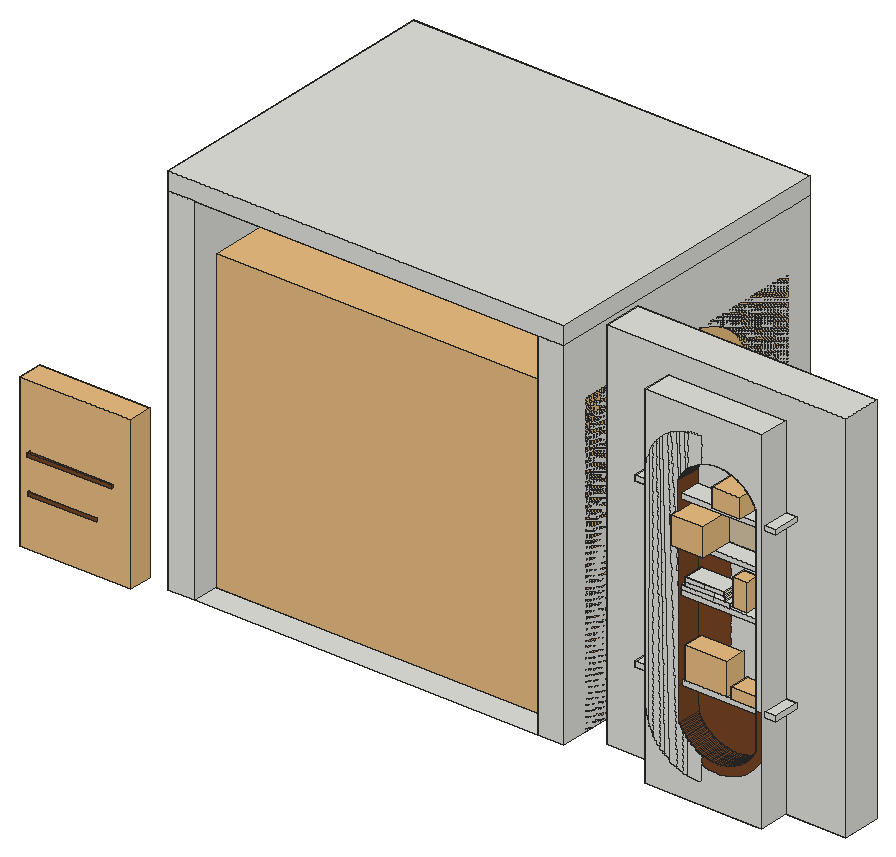
# SketchUp Ruby script. Lengths in inches.
U = 1.inch
M = Sketchup.active_model
def pt(a) = Geom::Point3d.new(a.map { |v| v * U })
def face(e, loops, mat)
  f = e.add_face(loops[0].map { |a| pt(a) })
  loops[1..].each { |l| e.add_face(l.map { |a| pt(a) }).erase! }
  f.material = f.back_material = mat if mat
  f
end
# faces: each face lists its corners as indices into pts; further lists are holes
def faces(e, pts, list, mat = nil) = list.each { |f| face(e, (f[0].is_a?(Array) ? f : [f]).map { |l| l.map { |i| pts[i] } }, mat) }
# xy, xz, yz: faces in a plane at the given z, y or x. An outline is a flat list of corners, or four numbers for a rectangle; further outlines are holes
def ring(l) = l.size == 4 ? [[l[0], l[1]], [l[2], l[1]], [l[2], l[3]], [l[0], l[3]]] : l.each_slice(2).to_a
def flat(e, list, mat, &to3) = list.each { |f| face(e, (f[0].is_a?(Array) ? f : [f]).map { |l| ring(l).map { |u, v| to3.(u, v) } }, mat) }
def xy(e, z, list, mat = nil) = flat(e, list, mat) { |x, y| [x, y, z] }
def xz(e, y, list, mat = nil) = flat(e, list, mat) { |x, z| [x, y, z] }
def yz(e, x, list, mat = nil) = flat(e, list, mat) { |y, z| [x, y, z] }
def lines(e, pts, list) = list.each { |a, b| e.add_line(pt(pts[a]), pt(pts[b])) }
# prism: a flat outline (further loops are holes) pulled along v
def prism(e, loops, v, mat = nil)
  f = face(e, loops, mat); d = Geom::Vector3d.new(v.map { |x| x * U })
  f.pushpull(f.normal.samedirection?(d) ? d.length : -d.length)
end
def box(e, o, s, mat = nil) = prism(e, [[o, [o[0] + s[0], o[1], o[2]], [o[0] + s[0], o[1] + s[1], o[2]], [o[0], o[1] + s[1], o[2]]]], [0, 0, s[2]], mat)
def at(x, y, z, deg = 0) = Geom::Transformation.translation(pt([x, y, z])) * Geom::Transformation.rotation(ORIGIN, Z_AXIS, deg.degrees)
def axes(o, x, y, z) = Geom::Transformation.new([*x, 0, *y, 0, *z, 0, *pt(o).to_a, 1])
def part(name) = M.definitions.add(name)
# library, detail: a bought-in or finely detailed component or shape, given as its bounding box
def library(name, o, s) = part(name).tap { |d| box(d.entities, o, s) }
def detail(e, o, s) = box(e.add_group.entities, o, s)
def put(e, d, t, mat = nil) = e.add_instance(d, t).tap { |i| i.material = mat if mat }
def group(e, t, mat = nil) = e.add_group.tap { |g| g.transformation = t; g.material = mat if mat }.entities
root = M.entities
M.materials.add("Douglas Fir, Staggered with Shadowgap (CXYQC8)").color = [216, 197, 167]
M.materials.add("[Color_000]").color = [255, 255, 255]
M.materials.add("[Color_D05]").color = [255, 242, 204]
M.materials.add("[Wood Veneer 01]").color = [120, 70, 37]
c1 = library("Sony_TV_KDL42W705B.skp\#1",[-24.34,-0.25,1.74],[48.68,2.34,28.26])
c2 = library("Component",[-53.76,-1.97,-0.51],[47.25,4.73,6.22])
c3 = library("Ring pendant light",[-446.05,-425.1,-51.8],[906.89,953.39,1136.48])
c4 = part("e7b7-889f-4641-7af6")
g1 = group(c4.entities,at(0,0,0))
g2 = group(g1,at(0,0,0))
put(g2,c3,axes([0,0,0],[39.37008,0,0],[0,39.37008,0],[0,0,39.37008]))
c5 = library("Plant_pot\#1",[-1.14,-1.38,0],[9.4,9.4,6.47])
c6 = library("Books+01+VRAY+ready",[65.64,68.87,0],[14.63,11.84,5.35])
c7 = part("Hardcover book")
xy(c7.entities,0,[[0.12,0.12,1.11,7.49]])
xy(c7.entities,0,[[0,0,0,7.57,0.12,7.57,0.12,0.12,1.11,0.12,1.11,7.57,1.22,7.57,1.22,0]],"[Color_000]")
xy(c7.entities,9.7,[[0.12,0.13,1.11,7.51]],"[Color_D05]")
xy(c7.entities,9.81,[[0,0.02,1.22,0.02,1.22,7.59,1.11,7.59,1.11,0.13,0.12,0.13,0.12,7.59,0,7.59]],"[Color_000]")
xz(c7.entities,0.13,[[0.12,9.7,1.11,9.81]],"[Color_000]")
yz(c7.entities,0,[[0,0,0.01,7.28,0.02,9.81,7.59,9.81,7.57,0]],"[Color_000]")
yz(c7.entities,0.12,[[0.12,0,7.49,0,7.51,9.7,0.13,9.7]])
yz(c7.entities,0.12,[[7.49,0,7.57,0,7.59,9.81,0.13,9.81,0.13,9.7,7.51,9.7]],"[Color_000]")
yz(c7.entities,1.11,[[0.12,0,0.13,9.7,7.51,9.7,7.49,0]])
yz(c7.entities,1.11,[[7.49,0,7.51,9.7,0.13,9.7,0.13,9.81,7.59,9.81,7.57,0]],"[Color_000]")
yz(c7.entities,1.22,[[0,0,7.57,0,7.59,9.81,0.02,9.81,0.01,7.28]])
p = [[1.22,0,0],[1.22,0.01,7.28],[0,0.01,7.28],[0,0,0],[1.11,0.12,0],[0.12,0.12,0],
  [0.12,0.13,9.7],[1.11,0.13,9.7],[1.11,7.49,0],[0.12,7.49,0],[0.12,7.51,9.7],[1.11,7.51,9.7],
  [0.12,7.57,0],[0,7.57,0],[0,7.59,9.81],[0.12,7.59,9.81],[1.22,7.57,0],[1.11,7.57,0],
  [1.11,7.59,9.81],[1.22,7.59,9.81],[0,0.02,9.81],[1.22,0.02,9.81]]
faces(c7.entities,p,[[0,1,2,3],[4,5,6,7],[12,13,14,15]])
faces(c7.entities,p,[[8,9,10,11]],"[Color_D05]")
faces(c7.entities,p,[[16,17,18,19],[20,2,1,21]],"[Color_000]")
c8 = part("Hardcover book \#1")
xy(c8.entities,0,[[0.12,0.12,1.11,6.86]])
xy(c8.entities,0,[[0,0,0,6.94,0.12,6.94,0.12,0.12,1.11,0.12,1.11,6.94,1.22,6.94,1.22,0]],"[Color_000]")
xy(c8.entities,9.46,[[0.12,0.13,1.11,6.88]],"[Color_D05]")
xy(c8.entities,9.57,[[0,0.02,1.22,0.02,1.22,6.96,1.11,6.96,1.11,0.13,0.12,0.13,0.12,6.96,0,6.96]],"[Color_000]")
xz(c8.entities,0.13,[[0.12,9.46,1.11,9.57]],"[Color_000]")
yz(c8.entities,0,[[0,0,0.01,4.79,0.02,9.57,6.96,9.57,6.94,0]])
yz(c8.entities,0.12,[[0.12,0,6.86,0,6.88,9.46,0.13,9.46]])
yz(c8.entities,0.12,[[6.86,0,6.94,0,6.96,9.57,0.13,9.57,0.13,9.46,6.88,9.46]],"[Color_000]")
yz(c8.entities,1.11,[[0.12,0,0.13,9.46,6.88,9.46,6.86,0]])
yz(c8.entities,1.11,[[6.86,0,6.88,9.46,0.13,9.46,0.13,9.57,6.96,9.57,6.94,0]],"[Color_000]")
yz(c8.entities,1.22,[[0,0,6.94,0,6.96,9.57,0.02,9.57,0.01,4.79]])
p = [[1.22,0,0],[1.22,0.01,4.79],[0,0.01,4.79],[0,0,0],[1.11,0.12,0],[0.12,0.12,0],
  [0.12,0.13,9.46],[1.11,0.13,9.46],[0.12,6.94,0],[0,6.94,0],[0,6.96,9.57],[0.12,6.96,9.57],
  [1.11,6.86,0],[0.12,6.86,0],[0.12,6.88,9.46],[1.11,6.88,9.46],[1.22,6.94,0],[1.11,6.94,0],
  [1.11,6.96,9.57],[1.22,6.96,9.57],[0,0.02,9.57],[1.22,0.02,9.57]]
faces(c8.entities,p,[[0,1,2,3],[4,5,6,7],[8,9,10,11],[20,2,1,21]])
faces(c8.entities,p,[[12,13,14,15]],"[Color_D05]")
faces(c8.entities,p,[[16,17,18,19]],"[Color_000]")
c9 = part("Hardcover book \#2")
xy(c9.entities,0,[[0.12,0.12,1.11,8.02]])
xy(c9.entities,0,[[0,0,0,8.1,0.12,8.1,0.12,0.12,1.11,0.12,1.11,8.1,1.22,8.1,1.22,0]],"[Color_000]")
xy(c9.entities,11.98,[[0.12,0.12,1.11,8.02]],"[Color_D05]")
xy(c9.entities,12.09,[[0,0,1.22,0,1.22,8.1,1.11,8.1,1.11,0.12,0.12,0.12,0.12,8.1,0,8.1]],"[Color_000]")
xz(c9.entities,0,[[0,0,1.22,7.96],[0,7.96,1.22,12.09]])
xz(c9.entities,0.12,[[0.12,0,1.11,11.98]])
xz(c9.entities,0.12,[[0.12,11.98,1.11,12.09]],"[Color_000]")
xz(c9.entities,8.02,[[0.12,0,1.11,11.98]],"[Color_D05]")
xz(c9.entities,8.1,[[0,0,0.12,12.09]])
xz(c9.entities,8.1,[[1.11,0,1.22,12.09]],"[Color_000]")
yz(c9.entities,0,[[0,0,8.1,12.09]])
yz(c9.entities,0.12,[[0.12,0,8.02,11.98]])
yz(c9.entities,0.12,[[8.02,0,8.1,0,8.1,12.09,0.12,12.09,0.12,11.98,8.02,11.98]],"[Color_000]")
yz(c9.entities,1.11,[[0.12,0,8.02,11.98]])
yz(c9.entities,1.11,[[8.02,0,8.02,11.98,0.12,11.98,0.12,12.09,8.1,12.09,8.1,0]],"[Color_000]")
yz(c9.entities,1.22,[[0,0,8.1,12.09]])
c10 = part("Stacked books")
put(c10.entities,c7,axes([15.01,10.96,2.78],[0,0,-1.13702],[0,-1.3536,0],[-1.3536,0,0]))
put(c10.entities,c8,axes([15.01,10.96,4.17],[0,0,-1.13702],[0,-1.3536,0],[-1.3536,0,0]))
put(c10.entities,c9,axes([16.36,10.96,1.39],[0,0,-1.13702],[0,-1.3536,0],[-1.3536,0,0]))
c11 = library("APARADOR+DE+LIVROS+CACHORRO",[95.16,10.21,2.45],[14.14,8.65,10.65])
c12 = library("Pot plante",[0,0,0],[98.24,106.18,82.98])
c13 = library("Group\#1",[0,0,0],[37,8,51])
c14 = library("Group\#10",[0,0,0],[110.17,20.41,51.91])
c15 = part("Group\#15")
box(c15.entities,[0,0,0],[47,9,1.66])
c16 = library("Group\#37",[0,0,0],[8.83,8.83,17.16])
detail(root,[42.01,15.87,0],[133,85,100.3125])
put(root,c1,at(104.17,100.77,52.78))
put(root,c2,axes([58.04,92.16,45.17],[0,0,-1],[-1,0,0],[0,1,0]))
put(root,c2,axes([156.21,94.16,49.36],[0,0,-1],[-1,0,0],[0,1,0]))
put(root,c4,axes([107.8,50.28,93.98],[0.00058,0,0],[0,0.00058,0],[0,0,0.00058]))
put(root,c5,at(228.14,5.31,90.75))
put(root,c6,axes([189.51,-39.46,34.75],[0.65,0,0],[0,0.65,0],[0,0,0.65]))
put(root,c10,at(231.86,16.27,61.75,-180))
put(root,c11,at(121.49,-4.9,32.31))
put(root,c12,axes([215.1875,1.31,76.7],[0.11,0,0],[0,0.11,0],[0,0,0.11]))
put(root,c13,at(-2.75,1,0))
g3 = group(root,at(0.2,0,28.33),"[Wood Veneer 01]")
prism(g3,[[[27.99,5.5625,0],[28.09,0.5625,0],[0.1,0,0],[0,5,0]]],[0,0,1.23])
g4 = group(root,at(-5.01,0.4375,16.27),"[Wood Veneer 01]")
xy(g4,0,[[5.1,0.1,5.01,4.56,28.01,5.02,28.09,0.5625]])
xy(g4,1.23,[[5.1,0.1,29.42,0.59,29.33,5.05,28.01,5.02,5.01,4.56]])
p = [[5.01,4.56,1.23],[5.01,4.56,0],[5.1,0.1,0],[5.1,0.1,1.23],[28.09,0.5625,0],[29.42,0.59,0],
  [29.42,0.59,1.23],[28.01,5.02,0],[28.01,5.02,1.23],[29.33,5.05,1.23]]
faces(g4,p,[[0,1,2,3],[2,4,5,6,3],[7,8,4],[4,8,9,5],[6,5,9],[8,7,1,0]])
g5 = group(root,at(166.01,6.87,0))
xy(g5,0,[[0,0,9,29.67],[0,77.14,9,103]])
xy(g5,120,[[0,0,9,103]])
xz(g5,0,[[0,0,9,120]])
xz(g5,29.67,[[0,0,9,82.3125]])
xz(g5,77.14,[[0,0,9,82.3125]])
xz(g5,103,[[0,0,9,120]])
yz(g5,0,[[0,0,0,120,94,120,94,0,77.14,0,77.14,82.3125,76.91,83.08,76.66,83.84,76.38,84.59,76.08,85.33,75.76,86.06,75.41,86.78,75.04,87.49,74.64,88.18,74.22,88.86,73.78,89.53,73.32,90.1875,72.84,90.82,72.34,91.45,71.82,92.05,71.28,92.64,70.72,93.21,70.14,93.76,69.54,94.3,68.93,94.8125,68.3,95.3,67.66,95.78,67,96.23,66.32,96.66,65.63,97.07,64.93,97.45,64.22,97.8125,63.5,98.15,62.76,98.47,62.02,98.76,61.26,99.03,60.5,99.27,59.73,99.49,58.95,99.68,58.17,99.85,57.39,99.99,56.59,100.11,55.8,100.2,55,100.26,54.2,100.3,53.4,100.3125,52.61,100.3,51.81,100.26,51.01,100.2,50.22,100.11,49.42,99.99,48.64,99.85,47.86,99.68,47.08,99.49,46.31,99.27,45.55,99.03,44.79,98.76,44.05,98.47,43.3125,98.15,42.59,97.8125,41.88,97.45,41.18,97.07,40.49,96.66,39.81,96.23,39.15,95.78,38.51,95.3,37.88,94.8125,37.27,94.3,36.67,93.76,36.09,93.21,35.53,92.64,34.99,92.05,34.47,91.45,33.97,90.82,33.49,90.1875,33.03,89.53,32.59,88.86,32.17,88.18,31.77,87.49,31.4,86.78,31.05,86.06,30.73,85.33,30.43,84.59,30.15,83.84,29.9,83.08,29.67,82.3125,29.67,0],[94,0,103,120]])
yz(g5,9,[[0,0,29.67,0,29.67,82.3125,29.9,83.08,30.15,83.84,30.43,84.59,30.73,85.33,31.05,86.06,31.4,86.78,31.77,87.49,32.17,88.18,32.59,88.86,33.03,89.53,33.49,90.1875,33.97,90.82,34.47,91.45,34.99,92.05,35.53,92.64,36.09,93.21,36.67,93.76,37.27,94.3,37.88,94.8125,38.51,95.3,39.15,95.78,39.81,96.23,40.49,96.66,41.18,97.07,41.88,97.45,42.59,97.8125,43.3125,98.15,44.05,98.47,44.79,98.76,45.55,99.03,46.31,99.27,47.08,99.49,47.86,99.68,48.64,99.85,49.42,99.99,50.22,100.11,51.01,100.2,51.81,100.26,52.61,100.3,53.4,100.3125,54.2,100.3,55,100.26,55.8,100.2,56.59,100.11,57.39,99.99,58.17,99.85,58.95,99.68,59.73,99.49,60.5,99.27,61.26,99.03,62.02,98.76,62.76,98.47,63.5,98.15,64.22,97.8125,64.93,97.45,65.63,97.07,66.32,96.66,67,96.23,67.66,95.78,68.3,95.3,68.93,94.8125,69.54,94.3,70.14,93.76,70.72,93.21,71.28,92.64,71.82,92.05,72.34,91.45,72.84,90.82,73.32,90.1875,73.78,89.53,74.22,88.86,74.64,88.18,75.04,87.49,75.41,86.78,75.76,86.06,76.08,85.33,76.38,84.59,76.66,83.84,76.91,83.08,77.14,82.3125,77.14,0,103,0,103,120,0,120]])
p = [[0,29.67,82.3125],[0,29.9,83.08],[9,29.9,83.08],[9,29.67,82.3125],[0,76.91,83.08],[0,77.14,82.3125],
  [9,77.14,82.3125],[9,76.91,83.08],[0,30.15,83.84],[9,30.15,83.84],[0,76.66,83.84],[9,76.66,83.84],
  [0,30.43,84.59],[9,30.43,84.59],[0,76.38,84.59],[9,76.38,84.59],[0,30.73,85.33],[9,30.73,85.33],
  [0,76.08,85.33],[9,76.08,85.33],[0,31.05,86.06],[9,31.05,86.06],[0,75.76,86.06],[9,75.76,86.06],
  [0,31.4,86.78],[9,31.4,86.78],[0,75.41,86.78],[9,75.41,86.78],[0,31.77,87.49],[9,31.77,87.49],
  [0,75.04,87.49],[9,75.04,87.49],[0,32.17,88.18],[9,32.17,88.18],[0,74.64,88.18],[9,74.64,88.18],
  [0,32.59,88.86],[9,32.59,88.86],[0,74.22,88.86],[9,74.22,88.86],[0,33.03,89.53],[9,33.03,89.53],
  [0,73.78,89.53],[9,73.78,89.53],[0,33.49,90.1875],[9,33.49,90.1875],[0,73.32,90.1875],[9,73.32,90.1875],
  [0,33.97,90.82],[9,33.97,90.82],[0,72.84,90.82],[9,72.84,90.82],[0,34.47,91.45],[9,34.47,91.45],
  [0,72.34,91.45],[9,72.34,91.45],[0,34.99,92.05],[9,34.99,92.05],[0,71.82,92.05],[9,71.82,92.05],
  [0,35.53,92.64],[9,35.53,92.64],[0,71.28,92.64],[9,71.28,92.64],[0,36.09,93.21],[9,36.09,93.21],
  [0,70.72,93.21],[9,70.72,93.21],[0,36.67,93.76],[9,36.67,93.76],[0,70.14,93.76],[9,70.14,93.76],
  [0,37.27,94.3],[9,37.27,94.3],[0,69.54,94.3],[9,69.54,94.3],[0,37.88,94.8125],[9,37.88,94.8125],
  [0,68.93,94.8125],[9,68.93,94.8125],[0,38.51,95.3],[9,38.51,95.3],[0,68.3,95.3],[9,68.3,95.3],
  [0,39.15,95.78],[9,39.15,95.78],[0,67.66,95.78],[9,67.66,95.78],[0,39.81,96.23],[9,39.81,96.23],
  [0,67,96.23],[9,67,96.23],[0,40.49,96.66],[9,40.49,96.66],[0,66.32,96.66],[9,66.32,96.66],
  [0,41.18,97.07],[9,41.18,97.07],[0,65.63,97.07],[9,65.63,97.07],[0,41.88,97.45],[9,41.88,97.45],
  [0,64.93,97.45],[9,64.93,97.45],[0,42.59,97.8125],[9,42.59,97.8125],[0,64.22,97.8125],[9,64.22,97.8125],
  [0,43.3125,98.15],[9,43.3125,98.15],[0,63.5,98.15],[9,63.5,98.15],[0,44.05,98.47],[9,44.05,98.47],
  [0,62.76,98.47],[9,62.76,98.47],[0,44.79,98.76],[9,44.79,98.76],[0,62.02,98.76],[9,62.02,98.76],
  [0,45.55,99.03],[9,45.55,99.03],[0,61.26,99.03],[9,61.26,99.03],[0,46.31,99.27],[9,46.31,99.27],
  [0,60.5,99.27],[9,60.5,99.27],[0,47.08,99.49],[9,47.08,99.49],[0,59.73,99.49],[9,59.73,99.49],
  [0,47.86,99.68],[9,47.86,99.68],[0,58.95,99.68],[9,58.95,99.68],[0,48.64,99.85],[9,48.64,99.85],
  [0,58.17,99.85],[9,58.17,99.85],[0,49.42,99.99],[9,49.42,99.99],[0,57.39,99.99],[9,57.39,99.99],
  [0,50.22,100.11],[9,50.22,100.11],[0,56.59,100.11],[9,56.59,100.11],[0,51.01,100.2],[9,51.01,100.2],
  [0,55.8,100.2],[9,55.8,100.2],[0,51.81,100.26],[9,51.81,100.26],[0,55,100.26],[9,55,100.26],
  [0,52.61,100.3],[9,52.61,100.3],[0,53.4,100.3125],[9,53.4,100.3125],[0,54.2,100.3],[9,54.2,100.3]]
faces(g5,p,[[0,1,2,3],[4,5,6,7],[1,8,9,2],[10,4,7,11],[8,12,13,9],[14,10,11,15],[12,16,17,13],[18,14,15,19],
  [16,20,21,17],[22,18,19,23],[20,24,25,21],[26,22,23,27],[24,28,29,25],[30,26,27,31],[28,32,33,29],[34,30,31,35],
  [32,36,37,33],[38,34,35,39],[36,40,41,37],[42,38,39,43],[40,44,45,41],[46,42,43,47],[44,48,49,45],[50,46,47,51],
  [48,52,53,49],[54,50,51,55],[52,56,57,53],[58,54,55,59],[56,60,61,57],[62,58,59,63],[60,64,65,61],[66,62,63,67],
  [64,68,69,65],[70,66,67,71],[68,72,73,69],[74,70,71,75],[72,76,77,73],[78,74,75,79],[76,80,81,77],[82,78,79,83],
  [80,84,85,81],[86,82,83,87],[84,88,89,85],[90,86,87,91],[88,92,93,89],[94,90,91,95],[92,96,97,93],[98,94,95,99],
  [96,100,101,97],[102,98,99,103],[100,104,105,101],[106,102,103,107],[104,108,109,105],[110,106,107,111],[108,112,113,109],[114,110,111,115],
  [112,116,117,113],[118,114,115,119],[116,120,121,117],[122,118,119,123],[120,124,125,121],[126,122,123,127],[124,128,129,125],[130,126,127,131],
  [128,132,133,129],[134,130,131,135],[132,136,137,133],[138,134,135,139],[136,140,141,137],[142,138,139,143],[140,144,145,141],[146,142,143,147],
  [144,148,149,145],[150,146,147,151],[148,152,153,149],[154,150,151,155],[152,156,157,153],[156,158,159,157],[158,160,161,159],[160,154,155,161]])
g6 = group(root,at(51.01,6.87,0))
xy(g6,0,[[0,0,115,9]])
g7 = group(root,at(42.01,6.87,0))
prism(g7,[[[9,25.2,0],[9,25.2,82.3125],[9,25.43,83.08],[9,25.68,83.84],[9,25.96,84.59],[9,26.26,85.33],[9,26.58,86.06],[9,26.93,86.78],[9,27.3,87.49],[9,27.7,88.18],[9,28.12,88.86],[9,28.56,89.53],[9,29.02,90.1875],[9,29.5,90.82],[9,30,91.45],[9,30.52,92.05],[9,31.0625,92.64],[9,31.625,93.21],[9,32.2,93.76],[9,32.8,94.3],[9,33.41,94.8125],[9,34.04,95.3],[9,34.69,95.78],[9,35.35,96.23],[9,36.02,96.66],[9,36.71,97.07],[9,37.41,97.45],[9,38.12,97.8125],[9,38.84,98.15],[9,39.58,98.47],[9,40.32,98.76],[9,41.08,99.03],[9,41.84,99.27],[9,42.61,99.49],[9,43.39,99.68],[9,44.17,99.85],[9,44.95,99.99],[9,45.75,100.11],[9,46.54,100.2],[9,47.34,100.26],[9,48.14,100.3],[9,48.9375,100.3125],[9,49.74,100.3],[9,50.53,100.26],[9,51.33,100.2],[9,52.125,100.11],[9,52.92,99.99],[9,53.7,99.85],[9,54.49,99.68],[9,55.26,99.49],[9,56.03,99.27],[9,56.79,99.03],[9,57.55,98.76],[9,58.29,98.47],[9,59.03,98.15],[9,59.75,97.8125],[9,60.46,97.45],[9,61.16,97.07],[9,61.85,96.66],[9,62.53,96.23],[9,63.1875,95.78],[9,63.83,95.3],[9,64.46,94.8125],[9,65.07,94.3],[9,65.67,93.76],[9,66.25,93.21],[9,66.81,92.64],[9,67.35,92.05],[9,67.87,91.45],[9,68.37,90.82],[9,68.85,90.1875],[9,69.31,89.53],[9,69.75,88.86],[9,70.17,88.18],[9,70.57,87.49],[9,70.9375,86.78],[9,71.29,86.06],[9,71.61,85.33],[9,71.91,84.59],[9,72.19,83.84],[9,72.44,83.08],[9,72.67,82.3125],[9,72.67,0],[9,103,0],[9,103,120],[9,0,120],[9,0,0]]],[-9,0,0])
g8 = group(root,at(51.01,100.87,0))
xy(g8,0,[[0,-1,1.83,0],[3,-1,4.83,0],[6,-1,7.83,0],[9,-1,10.83,0],[12,-1,13.83,0],
  [15,-1,16.83,0],[95.17,-1,97,0],[98.17,-1,100,0],[101.17,-1,103,0],[104.17,-1,106,0],
  [107.17,-1,109,0],[110.17,-1,112,0],[113.17,-1,115,0],[0,0,0,9,115,9,115,0,95.17,0,95.17,2,16.83,2,16.83,0]])
xy(g8,120,[[0,-1,1.83,0],[3,-1,4.83,0],[6,-1,7.83,0],[9,-1,10.83,0],[12,-1,13.83,0],
  [15,-1,16.83,0],[95.17,-1,97,0],[98.17,-1,100,0],[101.17,-1,103,0],[104.17,-1,106,0],
  [107.17,-1,109,0],[110.17,-1,112,0],[113.17,-1,115,0],[0,0,16.83,0,16.83,2,95.17,2,95.17,0,115,0,115,9,0,9]])
xz(g8,-1,[[0,0,1.83,120],[3,0,4.83,120],[6,0,7.83,120],[9,0,10.83,120],[12,0,13.83,120],
  [15,0,16.83,120],[95.17,0,97,120],[98.17,0,100,120],[101.17,0,103,120],[104.17,0,106,120],
  [107.17,0,109,120],[110.17,0,112,120],[113.17,0,115,120]])
xz(g8,0,[[0,0,1.83,120],[1.83,0,3,120],[3,0,4.83,120],[4.83,0,6,120],[6,0,7.83,120],
  [7.83,0,9,120],[9,0,10.83,120],[10.83,0,12,120],[12,0,13.83,120],[13.83,0,15,120],
  [15,0,16.83,120],[95.17,0,97,120],[97,0,98.17,120],[98.17,0,100,120],[100,0,101.17,120],
  [101.17,0,103,120],[103,0,104.17,120],[104.17,0,106,120],[106,0,107.17,120],[107.17,0,109,120],
  [109,0,110.17,120],[110.17,0,112,120],[112,0,113.17,120],[113.17,0,115,120]])
xz(g8,2,[[16.83,0,95.17,0,95.17,120,81.5,120,81.5,28,80.5,28,80.5,120,70.5,120,70.5,28,69.5,28,69.5,120,40.5,120,40.5,28,39.5,28,39.5,120,29.5,120,29.5,28,28.5,28,28.5,120,16.83,120],[28.5,28,29.5,120],[39.5,28,40.5,120],[69.5,28,70.5,120],[80.5,28,81.5,120]])
xz(g8,9,[[0,0,115,120]])
yz(g8,0,[[-1,0,0,120],[0,0,9,120]])
yz(g8,1.83,[[-1,0,0,120]])
yz(g8,3,[[-1,0,0,120]])
yz(g8,4.83,[[-1,0,0,120]])
yz(g8,6,[[-1,0,0,120]])
yz(g8,7.83,[[-1,0,0,120]])
yz(g8,9,[[-1,0,0,120]])
yz(g8,10.83,[[-1,0,0,120]])
yz(g8,12,[[-1,0,0,120]])
yz(g8,13.83,[[-1,0,0,120]])
yz(g8,15,[[-1,0,0,120]])
yz(g8,16.83,[[-1,0,0,120],[0,0,2,120]])
yz(g8,95.17,[[-1,0,0,120],[0,0,2,120]])
yz(g8,97,[[-1,0,0,120]])
yz(g8,98.17,[[-1,0,0,120]])
yz(g8,100,[[-1,0,0,120]])
yz(g8,101.17,[[-1,0,0,120]])
yz(g8,103,[[-1,0,0,120]])
yz(g8,104.17,[[-1,0,0,120]])
yz(g8,106,[[-1,0,0,120]])
yz(g8,107.17,[[-1,0,0,120]])
yz(g8,109,[[-1,0,0,120]])
yz(g8,110.17,[[-1,0,0,120]])
yz(g8,112,[[-1,0,0,120]])
yz(g8,113.17,[[-1,0,0,120]])
yz(g8,115,[[-1,0,0,120],[0,0,9,120]])
put(root,c14,at(52.85,84.85,11.96))
g9 = group(root,at(42.01,6.87,120))
xy(g9,-1,[[64.28,17.43,63.34,17.53,62.38,17.73,61.38,18.06,60.33,18.52,59.23,19.15,58.09,19.9375,56.93,20.91,55.76,22.08,54.61,23.4375,53.48,24.98,52.41,26.71,51.4,28.61,50.48,30.67,49.66,32.86,48.96,35.18,48.38,37.6,47.9375,40.11,47.64,42.67,47.48,45.27,47.47,47.875,47.6,50.48,47.89,53.05,48.31,55.56,48.87,57.99,49.55,60.33,50.36,62.54,51.26,64.62,52.26,66.54,53.32,68.3,54.44,69.87,55.6,71.26,56.77,72.45,57.93,73.45,59.07,74.27,60.17,74.91,61.23,75.4,62.24,75.75,63.21,75.97,64.15,76.08,65.07,76.08,66.01,75.99,66.97,75.78,67.97,75.46,69.03,74.99,70.12,74.37,71.26,73.58,72.42,72.6,73.59,71.4375,74.75,70.08,75.87,68.54,76.95,66.81,77.95,64.91,78.87,62.85,79.6875,60.65,80.39,58.33,80.97,55.91,81.41,53.41,81.72,50.85,81.875,48.25,81.88,45.64,81.75,43.04,81.47,40.47,81.04,37.96,80.48,35.53,79.8,33.19,79,30.98,78.09,28.9,77.1,26.97,76.03,25.22,74.91,23.65,73.76,22.26,72.59,21.07,71.42,20.07,70.28,19.25,69.18,18.6,68.12,18.12,67.11,17.77,66.15,17.55,65.21,17.44]])
xy(g9,0,[[[0,0,133,103],[63.63,3.46,66.08,3.48,68.52,3.76,70.9375,4.3125,73.31,5.125,75.64,6.2,77.9,7.52,80.07,9.08,82.16,10.87,84.13,12.89,85.98,15.11,87.71,17.53,89.29,20.13,90.72,22.89,91.98,25.8,93.08,28.84,94.01,31.99,94.75,35.23,95.31,38.55,95.68,41.91,95.86,45.3,95.84,48.7,95.64,52.09,95.24,55.45,94.66,58.76,93.89,61.98,92.9375,65.12,91.8125,68.14,90.52,71.03,89.07,73.77,87.47,76.35,85.72,78.74,83.85,80.9375,81.86,82.92,79.77,84.68,77.58,86.21,75.31,87.49,72.97,88.53,70.59,89.3,68.17,89.8125,65.72,90.0625,63.27,90.04,60.83,89.76,58.42,89.2,56.04,88.39,53.71,87.32,51.45,86,49.28,84.44,47.2,82.65,45.22,80.63,43.37,78.41,41.65,75.99,40.07,73.39,38.64,70.625,37.37,67.72,36.27,64.68,35.34,61.53,34.6,58.28,34.04,54.97,33.67,51.61,33.49,48.22,33.51,44.8125,33.71,41.42,34.11,38.07,34.7,34.76,35.47,31.53,36.42,28.4,37.54,25.375,38.83,22.48,40.28,19.74,41.89,17.17,43.63,14.78,45.5,12.58,47.49,10.6,49.59,8.84,51.77,7.31,54.04,6.03,56.38,4.99,58.76,4.22,61.18,3.7]],[[63.63,3.46,61.18,3.7,58.76,4.22,56.38,4.99,54.04,6.03,51.77,7.31,49.59,8.84,47.49,10.6,45.5,12.58,43.63,14.78,41.89,17.17,40.28,19.74,38.83,22.48,37.54,25.375,36.42,28.4,35.47,31.53,34.7,34.76,34.11,38.07,33.71,41.42,33.51,44.8125,33.49,48.22,33.67,51.61,34.04,54.97,34.6,58.28,35.34,61.53,36.27,64.68,37.37,67.72,38.64,70.625,40.07,73.39,41.65,75.99,43.37,78.41,45.22,80.63,47.2,82.65,49.28,84.44,51.45,86,53.71,87.32,56.04,88.39,58.42,89.2,60.83,89.76,63.27,90.04,65.72,90.0625,68.17,89.8125,70.59,89.3,72.97,88.53,75.31,87.49,77.58,86.21,79.77,84.68,81.86,82.92,83.85,80.9375,85.72,78.74,87.47,76.35,89.07,73.77,90.52,71.03,91.8125,68.14,92.9375,65.12,93.89,61.98,94.66,58.76,95.24,55.45,95.64,52.09,95.84,48.7,95.86,45.3,95.68,41.91,95.31,38.55,94.75,35.23,94.01,31.99,93.08,28.84,91.98,25.8,90.72,22.89,89.29,20.13,87.71,17.53,85.98,15.11,84.13,12.89,82.16,10.87,80.07,9.08,77.9,7.52,75.64,6.2,73.31,5.125,70.9375,4.3125,68.52,3.76,66.08,3.48],[63.6875,4.76,66,4.78,68.3,5.05,70.58,5.57,72.83,6.34,75.04,7.35,77.1875,8.61,79.27,10.1,81.26,11.82,83.16,13.76,84.95,15.91,86.62,18.25,88.15,20.77,89.54,23.45,90.77,26.28,91.85,29.25,92.75,32.32,93.47,35.49,94.02,38.73,94.38,42.02,94.56,45.33,94.54,48.66,94.34,51.98,93.95,55.26,93.38,58.49,92.63,61.64,91.7,64.7,90.61,67.65,89.35,70.46,87.9375,73.125,86.39,75.62,84.7,77.93,82.9,80.05,80.98,81.96,78.97,83.65,76.88,85.11,74.72,86.33,72.51,87.31,70.25,88.04,67.97,88.53,65.66,88.76,63.36,88.74,61.05,88.47,58.77,87.95,56.52,87.18,54.3125,86.17,52.16,84.91,50.08,83.42,48.09,81.7,46.1875,79.76,44.4,77.61,42.73,75.27,41.2,72.75,39.8125,70.07,38.58,67.23,37.51,64.27,36.6,61.2,35.88,58.03,35.33,54.79,34.97,51.5,34.8,48.18,34.81,44.86,35.01,41.54,35.4,38.26,35.97,35.03,36.72,31.875,37.65,28.8125,38.75,25.87,40,23.06,41.41,20.39,42.97,17.9,44.65,15.58,46.46,13.47,48.37,11.56,50.38,9.87,52.47,8.41,54.63,7.19,56.84,6.21,59.1,5.48,61.39,4.99]],[[63.6875,4.76,61.39,4.99,59.1,5.48,56.84,6.21,54.63,7.19,52.47,8.41,50.38,9.87,48.37,11.56,46.46,13.47,44.65,15.58,42.97,17.9,41.41,20.39,40,23.06,38.75,25.87,37.65,28.8125,36.72,31.875,35.97,35.03,35.4,38.26,35.01,41.54,34.81,44.86,34.8,48.18,34.97,51.5,35.33,54.79,35.88,58.03,36.6,61.2,37.51,64.27,38.58,67.23,39.8125,70.07,41.2,72.75,42.73,75.27,44.4,77.61,46.1875,79.76,48.09,81.7,50.08,83.42,52.16,84.91,54.3125,86.17,56.52,87.18,58.77,87.95,61.05,88.47,63.36,88.74,65.66,88.76,67.97,88.53,70.25,88.04,72.51,87.31,74.72,86.33,76.88,85.11,78.97,83.65,80.98,81.96,82.9,80.05,84.7,77.93,86.39,75.62,87.9375,73.125,89.35,70.46,90.61,67.65,91.7,64.7,92.63,61.64,93.38,58.49,93.95,55.26,94.34,51.98,94.54,48.66,94.56,45.33,94.38,42.02,94.02,38.73,93.47,35.49,92.75,32.32,91.85,29.25,90.77,26.28,89.54,23.45,88.15,20.77,86.62,18.25,84.95,15.91,83.16,13.76,81.26,11.82,79.27,10.1,77.1875,8.61,75.04,7.35,72.83,6.34,70.58,5.57,68.3,5.05,66,4.78],[64.28,17.43,65.21,17.44,66.15,17.55,67.11,17.77,68.12,18.12,69.18,18.6,70.28,19.25,71.42,20.07,72.59,21.07,73.76,22.26,74.91,23.65,76.03,25.22,77.1,26.97,78.09,28.9,79,30.98,79.8,33.19,80.48,35.53,81.04,37.96,81.47,40.47,81.75,43.04,81.88,45.64,81.875,48.25,81.72,50.85,81.41,53.41,80.97,55.91,80.39,58.33,79.6875,60.65,78.87,62.85,77.95,64.91,76.95,66.81,75.87,68.54,74.75,70.08,73.59,71.4375,72.42,72.6,71.26,73.58,70.12,74.37,69.03,74.99,67.97,75.46,66.97,75.78,66.01,75.99,65.07,76.08,64.15,76.08,63.21,75.97,62.24,75.75,61.23,75.4,60.17,74.91,59.07,74.27,57.93,73.45,56.77,72.45,55.6,71.26,54.44,69.87,53.32,68.3,52.26,66.54,51.26,64.62,50.36,62.54,49.55,60.33,48.87,57.99,48.31,55.56,47.89,53.05,47.6,50.48,47.47,47.875,47.48,45.27,47.64,42.67,47.9375,40.11,48.38,37.6,48.96,35.18,49.66,32.86,50.48,30.67,51.4,28.61,52.41,26.71,53.48,24.98,54.61,23.4375,55.76,22.08,56.93,20.91,58.09,19.9375,59.23,19.15,60.33,18.52,61.38,18.06,62.38,17.73,63.34,17.53]]])
xy(g9,6,[[0,0,133,103]])
xz(g9,0,[[0,0,133,6]])
xz(g9,76.08,[[64.15,-1,65.07,0]])
xz(g9,103,[[0,0,133,6]])
yz(g9,0,[[0,0,103,6]])
yz(g9,133,[[0,0,103,6]])
p = [[64.28,17.43,0],[63.34,17.53,0],[63.34,17.53,-1],[64.28,17.43,-1],[65.21,17.44,0],[65.21,17.44,-1],
  [66.15,17.55,0],[66.15,17.55,-1],[62.38,17.73,0],[62.38,17.73,-1],[67.11,17.77,0],[67.11,17.77,-1],
  [61.38,18.06,0],[61.38,18.06,-1],[68.12,18.12,0],[68.12,18.12,-1],[60.33,18.52,0],[60.33,18.52,-1],
  [69.18,18.6,0],[69.18,18.6,-1],[59.23,19.15,0],[59.23,19.15,-1],[70.28,19.25,0],[70.28,19.25,-1],
  [58.09,19.9375,0],[58.09,19.9375,-1],[71.42,20.07,0],[71.42,20.07,-1],[56.93,20.91,0],[56.93,20.91,-1],
  [72.59,21.07,0],[72.59,21.07,-1],[55.76,22.08,0],[55.76,22.08,-1],[73.76,22.26,0],[73.76,22.26,-1],
  [54.61,23.4375,0],[54.61,23.4375,-1],[74.91,23.65,0],[74.91,23.65,-1],[53.48,24.98,0],[53.48,24.98,-1],
  [76.03,25.22,0],[76.03,25.22,-1],[52.41,26.71,0],[52.41,26.71,-1],[77.1,26.97,0],[77.1,26.97,-1],
  [51.4,28.61,0],[51.4,28.61,-1],[78.09,28.9,0],[78.09,28.9,-1],[50.48,30.67,0],[50.48,30.67,-1],
  [79,30.98,0],[79,30.98,-1],[49.66,32.86,0],[49.66,32.86,-1],[79.8,33.19,0],[79.8,33.19,-1],
  [48.96,35.18,0],[48.96,35.18,-1],[80.48,35.53,0],[80.48,35.53,-1],[48.38,37.6,0],[48.38,37.6,-1],
  [81.04,37.96,0],[81.04,37.96,-1],[47.9375,40.11,0],[47.9375,40.11,-1],[81.47,40.47,0],[81.47,40.47,-1],
  [47.64,42.67,0],[47.64,42.67,-1],[81.75,43.04,0],[81.75,43.04,-1],[47.48,45.27,0],[47.48,45.27,-1],
  [81.88,45.64,0],[81.88,45.64,-1],[47.47,47.875,0],[47.47,47.875,-1],[81.875,48.25,0],[81.875,48.25,-1],
  [47.6,50.48,0],[47.6,50.48,-1],[81.72,50.85,0],[81.72,50.85,-1],[47.89,53.05,0],[47.89,53.05,-1],
  [81.41,53.41,0],[81.41,53.41,-1],[48.31,55.56,0],[48.31,55.56,-1],[80.97,55.91,0],[80.97,55.91,-1],
  [48.87,57.99,0],[48.87,57.99,-1],[80.39,58.33,0],[80.39,58.33,-1],[49.55,60.33,0],[49.55,60.33,-1],
  [79.6875,60.65,0],[79.6875,60.65,-1],[50.36,62.54,0],[50.36,62.54,-1],[78.87,62.85,0],[78.87,62.85,-1],
  [51.26,64.62,0],[51.26,64.62,-1],[77.95,64.91,0],[77.95,64.91,-1],[52.26,66.54,0],[52.26,66.54,-1],
  [76.95,66.81,0],[76.95,66.81,-1],[53.32,68.3,0],[53.32,68.3,-1],[75.87,68.54,0],[75.87,68.54,-1],
  [54.44,69.87,0],[54.44,69.87,-1],[74.75,70.08,0],[74.75,70.08,-1],[55.6,71.26,0],[55.6,71.26,-1],
  [73.59,71.4375,0],[73.59,71.4375,-1],[56.77,72.45,0],[56.77,72.45,-1],[72.42,72.6,0],[72.42,72.6,-1],
  [57.93,73.45,0],[57.93,73.45,-1],[71.26,73.58,0],[71.26,73.58,-1],[59.07,74.27,0],[59.07,74.27,-1],
  [70.12,74.37,0],[70.12,74.37,-1],[60.17,74.91,0],[60.17,74.91,-1],[69.03,74.99,0],[69.03,74.99,-1],
  [61.23,75.4,0],[61.23,75.4,-1],[67.97,75.46,0],[67.97,75.46,-1],[62.24,75.75,0],[62.24,75.75,-1],
  [66.97,75.78,0],[66.97,75.78,-1],[63.21,75.97,0],[63.21,75.97,-1],[66.01,75.99,0],[66.01,75.99,-1],
  [64.15,76.08,0],[64.15,76.08,-1],[65.07,76.08,0],[65.07,76.08,-1]]
faces(g9,p,[[0,1,2,3],[4,0,3,5],[6,4,5,7],[1,8,9,2],[10,6,7,11],[8,12,13,9],[14,10,11,15],[12,16,17,13],
  [18,14,15,19],[16,20,21,17],[22,18,19,23],[20,24,25,21],[26,22,23,27],[24,28,29,25],[30,26,27,31],[28,32,33,29],
  [34,30,31,35],[32,36,37,33],[38,34,35,39],[36,40,41,37],[42,38,39,43],[40,44,45,41],[46,42,43,47],[44,48,49,45],
  [50,46,47,51],[48,52,53,49],[54,50,51,55],[52,56,57,53],[58,54,55,59],[56,60,61,57],[62,58,59,63],[60,64,65,61],
  [66,62,63,67],[64,68,69,65],[70,66,67,71],[68,72,73,69],[74,70,71,75],[72,76,77,73],[78,74,75,79],[76,80,81,77],
  [82,78,79,83],[80,84,85,81],[86,82,83,87],[84,88,89,85],[90,86,87,91],[88,92,93,89],[94,90,91,95],[92,96,97,93],
  [98,94,95,99],[96,100,101,97],[102,98,99,103],[100,104,105,101],[106,102,103,107],[104,108,109,105],[110,106,107,111],[108,112,113,109],
  [114,110,111,115],[112,116,117,113],[118,114,115,119],[116,120,121,117],[122,118,119,123],[120,124,125,121],[126,122,123,127],[124,128,129,125],
  [130,126,127,131],[128,132,133,129],[134,130,131,135],[132,136,137,133],[138,134,135,139],[136,140,141,137],[142,138,139,143],[140,144,145,141],
  [146,142,143,147],[144,148,149,145],[150,146,147,151],[148,152,153,149],[154,150,151,155],[152,156,157,153],[158,154,155,159]])
put(root,c15,at(200.13,5.31,89.09))
g10 = group(root,at(200.13,5.31,60.09))
box(g10,[15.37,0,0],[25.89,9,1.66])
put(root,c15,at(200.13,5.31,33.09))
g11 = group(root,at(183.39,4.31,0))
xy(g11,0,[[20.74,0,20.74,10,0,10,0,23,80,23,80,10,58,10,58,0],[58,0,60,10]])
xy(g11,118.33,[[20.74,0,60,10]])
xy(g11,126,[[0,10,80,23]])
xz(g11,0,[[20.74,0,60,0,60,20.26,59.82,19.93,59.57,19.49,59.03,18.65,58.74,18.24,58.4375,17.84,58.125,17.45,57.8,17.06,57.47,16.69,57.12,16.33,56.4,15.63,56.02,15.3,55.64,14.98,55.24,14.67,54.84,14.38,54.43,14.09,54,13.82,53.58,13.5625,53.14,13.31,52.7,13.08,52.25,12.86,51.79,12.65,51.33,12.46,50.86,12.28,50.39,12.11,49.91,11.96,49.43,11.82,48.94,11.7,48.45,11.59,47.96,11.49,47.47,11.41,46.97,11.34,46.47,11.29,45.47,11.23,44.47,11.23,43.47,11.29,42.97,11.34,42.47,11.41,41.98,11.49,41.49,11.59,41,11.7,40.51,11.82,40.03,11.96,39.74,12.05,39.74,6.78,39.375,6.76,39.01,6.76,38.64,6.75,38.28,6.76,37.91,6.77,37.55,6.79,37.18,6.82,36.82,6.86,36.45,6.9,36.09,6.95,35.37,7.07,35.2,7.11,35.01,7.14,34.65,7.22,34.3,7.3125,33.94,7.41,33.24,7.61,32.9,7.73,32.55,7.85,32.21,7.98,31.53,8.26,31.2,8.41,30.54,8.73,30.22,8.9,29.58,9.26,29.27,9.45,28.65,9.85,28.05,10.27,27.76,10.49,27.47,10.72,27.19,10.95,26.91,11.1875,26.64,11.43,26.37,11.68,26.11,11.93,25.85,12.19,25.35,12.73,25.11,13,24.87,13.28,24.64,13.57,24.42,13.85,24.2,14.15,23.78,14.75,23.58,15.05,23.38,15.36,22.84,16.32,22.67,16.64,22.51,16.97,22.36,17.3,22.21,17.64,22.07,17.97,21.93,18.32,21.8,18.66,21.68,19,21.46,19.7,21.37,20.05,21.27,20.41,21.1875,20.76,21.11,21.12,21.04,21.48,20.92,22.2,20.875,22.57,20.83,22.93,20.8,23.29,20.77,23.66,20.76,24.02,20.74,24.39,20.74,24.76],[38.64,6.75,39.01,6.76,39.375,6.76,39.74,6.78,39.74,15.18,39.7,15.19,39.32,15.35,38.94,15.53,38.57,15.71,38.2,15.9,37.84,16.11,37.49,16.32,37.14,16.55,36.8,16.78,36.46,17.03,35.82,17.55,35.5,17.82,35.2,18.11,35.2,7.11,35.37,7.07,36.09,6.95,36.45,6.9,36.82,6.86,37.18,6.82,37.55,6.79,37.91,6.77,38.28,6.76],[35.2,7.11,35.2,18.11,34.91,18.4,34.62,18.7,34.34,19.01,34.07,19.33,33.82,19.65,33.57,19.98,33.33,20.32,33.59,7.51,33.94,7.41,34.3,7.3125,34.65,7.22,35.01,7.14],[33.59,7.51,33.33,20.32,33.1,20.67,32.88,21.02,32.67,21.38,32.47,21.75,32.29,22.12,32.24,33.09,32.12,58.51,29.58,108.51,29.27,108.32,28.96,108.125,28.65,107.92,28.35,107.71,31.53,8.26,32.21,7.98,32.55,7.85,32.9,7.73,33.24,7.61],[31.53,8.26,28.35,107.71,28.05,107.5,27.76,107.28,27.47,107.05,27.19,106.82,26.91,106.58,29.27,9.45,29.58,9.26,30.22,8.9,30.54,8.73,31.2,8.41],
  [29.27,9.45,26.91,106.58,26.64,106.34,26.37,106.09,26.11,105.84,25.85,105.58,25.6,105.3125,27.47,10.72,27.76,10.49,28.05,10.27,28.65,9.85],[27.47,10.72,25.6,105.3125,25.35,105.04,25.11,104.77,24.87,104.49,24.64,104.2,25.6,12.46,25.85,12.19,26.11,11.93,26.37,11.68,26.64,11.43,26.91,11.1875,27.19,10.95],[25.6,12.46,24.64,104.2,24.42,103.92,24.2,103.62,23.78,103.02,23.58,102.72,23.58,15.05,23.78,14.75,24.2,14.15,24.42,13.85,24.64,13.57,24.87,13.28,25.11,13,25.35,12.73],[23.58,15.05,23.58,102.72,23.38,102.41,22.84,101.45,22.67,101.125,22.51,100.8,22.21,17.64,22.36,17.3,22.51,16.97,22.67,16.64,22.84,16.32,23.38,15.36],[22.21,17.64,22.51,100.8,22.36,100.47,22.21,100.13,21.93,99.45,21.8,99.11,21.68,98.77,21.46,98.07,21.37,97.72,21.27,97.36,21.1875,97.01,21.11,96.65,21.04,96.29,20.92,95.57,20.875,95.2,20.83,94.84,20.8,94.48,20.77,94.11,20.76,93.74,20.75,93.47,20.74,93.38,20.74,24.39,20.76,24.02,20.77,23.66,20.8,23.29,20.83,22.93,20.875,22.57,20.92,22.2,21.04,21.48,21.11,21.12,21.1875,20.76,21.27,20.41,21.37,20.05,21.46,19.7,21.68,19,21.8,18.66,21.93,18.32,22.07,17.97],
  [58,34.78,60,34.78,60,118.33,20.74,118.33,20.74,94.89,20.75,93.47,20.76,93.74,20.77,94.11,20.8,94.48,20.83,94.84,20.875,95.2,20.92,95.57,21.04,96.29,21.11,96.65,21.1875,97.01,21.27,97.36,21.37,97.72,21.46,98.07,21.68,98.77,21.8,99.11,21.93,99.45,22.21,100.13,22.36,100.47,22.51,100.8,22.67,101.125,22.84,101.45,23.38,102.41,23.58,102.72,23.78,103.02,24.2,103.62,24.42,103.92,24.64,104.2,24.87,104.49,25.11,104.77,25.35,105.04,25.6,105.3125,25.85,105.58,26.11,105.84,26.37,106.09,26.64,106.34,26.91,106.58,27.19,106.82,27.47,107.05,27.76,107.28,28.05,107.5,28.65,107.92,28.96,108.125,29.27,108.32,29.58,108.51,30.22,108.87,30.54,109.04,31.2,109.36,31.53,109.51,32.21,109.79,32.55,109.92,32.9,110.04,33.24,110.16,33.94,110.36,34.3,110.46,34.65,110.55,35.37,110.7,36.09,110.82,36.45,110.87,36.82,110.91,37.18,110.95,37.55,110.98,37.91,111,38.28,111.01,38.64,111.02,39.01,111.01,39.74,110.99,39.74,102.59,40.09,102.73,40.48,102.86,40.88,102.99,41.68,103.21,42.09,103.3,42.49,103.38,43.31,103.5,43.73,103.54,44.14,103.57,44.56,103.59,44.97,103.6,45.39,103.59,45.8,103.57,46.22,103.54,46.63,103.5,47.45,103.38,47.86,103.3,48.26,103.21,48.66,103.1,49.0625,102.99,49.46,102.86,49.85,102.73,50.24,102.58,50.62,102.42,51,102.24,51.37,102.0625,51.74,101.87,52.46,101.45,52.8,101.22,53.15,100.99,53.48,100.74,53.81,100.48,54.13,100.22,54.4375,99.94,54.74,99.66,55.04,99.37,55.32,99.07,55.6,98.76,55.87,98.44,56.13,98.12,56.375,97.79,56.62,97.45,56.84,97.1,57.0625,96.75,57.27,96.39,57.47,96.02,57.66,95.65,58,94.89],[32.12,58.51,31.95,94.89,31.2,109.36,30.54,109.04,30.22,108.87,29.58,108.51],[20.74,93.01,20.74,93.38,20.75,93.47,20.74,94.89],[31.95,94.89,32.11,95.27,32.29,95.65,32.47,96.02,32.67,96.39,32.55,109.92,32.21,109.79,31.53,109.51,31.2,109.36],[32.67,96.39,32.88,96.75,33.1,97.1,33.33,97.45,33.57,97.79,33.82,98.12,34.07,98.44,33.94,110.36,33.24,110.16,32.9,110.04,32.55,109.92],
  [34.07,98.44,34.34,98.76,34.62,99.07,34.91,99.37,35.01,99.47,35.01,110.625,34.65,110.55,34.3,110.46,33.94,110.36],[35.01,99.47,35.2,99.66,35.5,99.94,35.82,100.22,36.46,100.74,36.8,100.99,37.14,101.22,37.49,101.45,37.84,101.66,38.2,101.87,38.57,102.0625,38.94,102.24,39.32,102.42,39.7,102.58,39.74,102.59,39.74,110.99,39.01,111.01,38.64,111.02,38.28,111.01,37.91,111,37.55,110.98,37.18,110.95,36.82,110.91,36.45,110.87,36.09,110.82,35.37,110.7,35.01,110.625]])
xz(g11,0,[[44.47,11.23,45.47,11.23,46.47,11.29,46.97,11.34,47.47,11.41,47.96,11.49,48.45,11.59,48.94,11.7,49.43,11.82,49.91,11.96,50.39,12.11,50.86,12.28,51.33,12.46,51.79,12.65,52.25,12.86,52.7,13.08,53.14,13.31,53.58,13.5625,54,13.82,54.43,14.09,54.84,14.38,55.24,14.67,55.64,14.98,56.02,15.3,56.4,15.63,57.12,16.33,57.47,16.69,57.8,17.06,58.125,17.45,58.4375,17.84,58.74,18.24,59.03,18.65,59.57,19.49,59.82,19.93,60,20.26,60,34.78,58,34.78,58,22.875,57.83,22.49,57.66,22.12,57.47,21.75,57.27,21.38,57.0625,21.02,56.84,20.67,56.62,20.32,56.375,19.98,56.13,19.65,55.87,19.33,55.6,19.01,55.32,18.7,55.04,18.4,54.74,18.11,54.4375,17.82,54.13,17.55,53.81,17.29,53.48,17.03,53.15,16.78,52.8,16.55,52.46,16.32,51.74,15.9,51.37,15.71,51,15.53,50.62,15.35,50.24,15.19,49.85,15.04,49.46,14.91,49.0625,14.78,48.66,14.66,48.26,14.5625,47.86,14.47,47.45,14.39,47.04,14.32,46.63,14.27,46.22,14.23,45.8,14.2,45.39,14.18,44.97,14.17,44.56,14.18,44.14,14.2,43.73,14.23,43.31,14.27,42.9,14.32,42.49,14.39,42.09,14.47,41.68,14.5625,41.28,14.66,40.88,14.78,40.48,14.91,40.09,15.04,39.74,15.18,39.74,12.05,40.03,11.96,40.51,11.82,41,11.7,41.49,11.59,41.98,11.49,42.47,11.41,42.97,11.34,43.47,11.29]],"[Wood Veneer 01]")
xz(g11,8,[[32.32,14.22,43.31,14.27,42.9,14.32,42.49,14.39,42.09,14.47,41.68,14.5625,41.28,14.66,40.88,14.78,40.48,14.91,40.09,15.04,39.74,15.18,39.7,15.19,39.32,15.35,38.94,15.53,38.57,15.71,38.2,15.9,37.84,16.11,37.49,16.32,37.14,16.55,36.8,16.78,36.46,17.03,35.82,17.55,35.5,17.82,35.2,18.11,34.91,18.4,34.62,18.7,34.34,19.01,34.07,19.33,33.82,19.65,33.57,19.98,33.33,20.32,33.1,20.67,32.88,21.02,32.67,21.38,32.47,21.75,32.29,22.12],[43.23,33.09,58,33.09,58,76.7,32.03,76.7,32.03,76.58,32.04,75.04,43.03,75.09],[31.97,89.09,58,89.09,58,94.89,57.66,95.65,57.47,96.02,57.27,96.39,57.0625,96.75,56.84,97.1,56.62,97.45,56.375,97.79,56.13,98.12,55.87,98.44,55.6,98.76,55.32,99.07,55.04,99.37,54.74,99.66,54.4375,99.94,54.13,100.22,53.81,100.48,53.48,100.74,53.15,100.99,52.8,101.22,52.46,101.45,51.74,101.87,51.37,102.0625,51,102.24,50.62,102.42,50.24,102.58,49.85,102.73,49.46,102.86,49.0625,102.99,48.66,103.1,48.26,103.21,47.86,103.3,47.45,103.38,46.63,103.5,46.22,103.54,45.8,103.57,45.39,103.59,44.97,103.6,44.56,103.59,44.14,103.57,43.73,103.54,43.31,103.5,42.49,103.38,42.09,103.3,41.68,103.21,40.88,102.99,40.48,102.86,40.09,102.73,39.74,102.59,39.7,102.58,39.32,102.42,38.94,102.24,38.57,102.0625,38.2,101.87,37.84,101.66,37.49,101.45,37.14,101.22,36.8,100.99,36.46,100.74,35.82,100.22,35.5,99.94,35.2,99.66,34.91,99.37,34.62,99.07,34.34,98.76,34.07,98.44,33.82,98.12,33.57,97.79,33.33,97.45,33.1,97.1,32.88,96.75,32.67,96.39,32.47,96.02,32.29,95.65,32.11,95.27,31.95,94.89]])
xz(g11,8,[[32.03,76.7,58,76.7,58,89.09,31.97,89.09]],"Douglas Fir, Staggered with Shadowgap (CXYQC8)")
xz(g11,8,[[44.97,14.17,45.39,14.18,45.8,14.2,46.22,14.23,46.63,14.27,47.04,14.32,47.45,14.39,47.86,14.47,48.26,14.5625,48.66,14.66,49.0625,14.78,49.46,14.91,49.85,15.04,50.24,15.19,50.62,15.35,51,15.53,51.37,15.71,51.74,15.9,52.46,16.32,52.8,16.55,53.15,16.78,53.48,17.03,53.81,17.29,54.13,17.55,54.4375,17.82,54.74,18.11,55.04,18.4,55.32,18.7,55.6,19.01,55.87,19.33,56.13,19.65,56.375,19.98,56.62,20.32,56.84,20.67,57.0625,21.02,57.27,21.38,57.47,21.75,57.66,22.12,57.83,22.49,58,22.875,58,33.09,43.23,33.09,43.03,75.09,32.04,75.04,32.24,33.09,32.29,22.12,32.47,21.75,32.67,21.38,32.88,21.02,33.1,20.67,33.33,20.32,33.57,19.98,33.82,19.65,34.07,19.33,34.34,19.01,34.62,18.7,34.91,18.4,35.2,18.11,35.5,17.82,35.82,17.55,36.46,17.03,36.8,16.78,37.14,16.55,37.49,16.32,37.84,16.11,38.2,15.9,38.57,15.71,38.94,15.53,39.32,15.35,39.7,15.19,39.74,15.18,40.09,15.04,40.48,14.91,40.88,14.78,41.28,14.66,41.68,14.5625,42.09,14.47,42.49,14.39,42.9,14.32,43.31,14.27,43.73,14.23,44.14,14.2,44.56,14.18]],"[Wood Veneer 01]")
xz(g11,10,[[0,0,20.74,0,20.74,118.33,60,118.33,60,0,80,0,80,126,0,126],[58,0,60,118.33]])
xz(g11,23,[[0,0,80,126]])
yz(g11,0,[[10,0,23,126]])
yz(g11,20.74,[[0,0,10,118.33]])
yz(g11,58,[[0,22.875,8,33.09],[0,33.09,8,94.89]],"[Wood Veneer 01]")
yz(g11,60,[[0,0,10,118.33]])
yz(g11,80,[[10,0,23,126]])
p = [[43.31,0,14.27],[43.73,0,14.23],[43.73,8,14.23],[43.31,8,14.27],[44.14,0,14.2],[44.14,8,14.2],
  [44.56,0,14.18],[44.56,8,14.18],[44.97,0,14.17],[44.97,8,14.17],[45.39,0,14.18],[45.39,8,14.18],
  [45.8,0,14.2],[45.8,8,14.2],[46.22,0,14.23],[46.22,8,14.23],[46.63,0,14.27],[46.63,8,14.27],
  [42.49,0,14.39],[42.9,0,14.32],[42.9,8,14.32],[42.49,8,14.39],[47.04,0,14.32],[47.04,8,14.32],
  [47.45,0,14.39],[47.45,8,14.39],[42.09,0,14.47],[42.09,8,14.47],[47.86,0,14.47],[47.86,8,14.47],
  [41.68,0,14.5625],[41.68,8,14.5625],[48.26,0,14.5625],[48.26,8,14.5625],[41.28,0,14.66],[41.28,8,14.66],
  [48.66,0,14.66],[48.66,8,14.66],[40.88,0,14.78],[40.88,8,14.78],[49.0625,0,14.78],[49.0625,8,14.78],
  [40.48,0,14.91],[40.48,8,14.91],[49.46,0,14.91],[49.46,8,14.91],[40.09,0,15.04],[40.09,8,15.04],
  [49.85,0,15.04],[49.85,8,15.04],[39.7,0,15.19],[39.74,0,15.18],[39.74,8,15.18],[39.7,8,15.19],
  [50.24,0,15.19],[50.24,8,15.19],[39.32,0,15.35],[39.32,8,15.35],[50.62,0,15.35],[50.62,8,15.35],
  [38.94,0,15.53],[38.94,8,15.53],[51,0,15.53],[51,8,15.53],[38.57,0,15.71],[38.57,8,15.71],
  [51.37,0,15.71],[51.37,8,15.71],[38.2,0,15.9],[38.2,8,15.9],[51.74,0,15.9],[51.74,8,15.9],
  [37.84,0,16.11],[37.84,8,16.11],[52.1,0,16.11],[52.1,8,16.11],[37.49,0,16.32],[37.49,8,16.32],
  [52.46,0,16.32],[52.46,8,16.32],[37.14,0,16.55],[37.14,8,16.55],[52.8,0,16.55],[52.8,8,16.55],
  [36.8,0,16.78],[36.8,8,16.78],[53.15,0,16.78],[53.15,8,16.78],[36.46,0,17.03],[36.46,8,17.03],
  [53.48,0,17.03],[53.48,8,17.03],[36.14,0,17.29],[36.14,8,17.29],[53.81,0,17.29],[53.81,8,17.29],
  [35.82,0,17.55],[35.82,8,17.55],[54.13,0,17.55],[54.13,8,17.55],[35.5,0,17.82],[35.5,8,17.82],
  [54.4375,0,17.82],[54.4375,8,17.82],[35.2,0,18.11],[35.2,8,18.11],[54.74,0,18.11],[54.74,8,18.11],
  [34.91,0,18.4],[34.91,8,18.4],[55.04,0,18.4],[55.04,8,18.4],[34.62,0,18.7],[34.62,8,18.7],
  [55.32,0,18.7],[55.32,8,18.7],[34.34,0,19.01],[34.34,8,19.01],[55.6,0,19.01],[55.6,8,19.01],
  [34.07,0,19.33],[34.07,8,19.33],[55.87,0,19.33],[55.87,8,19.33],[33.82,0,19.65],[33.82,8,19.65],
  [56.13,0,19.65],[56.13,8,19.65],[33.57,0,19.98],[33.57,8,19.98],[56.375,0,19.98],[56.375,8,19.98],
  [33.33,0,20.32],[33.33,8,20.32],[56.62,0,20.32],[56.62,8,20.32],[33.1,0,20.67],[33.1,8,20.67],
  [56.84,0,20.67],[56.84,8,20.67],[32.88,0,21.02],[32.88,8,21.02],[57.0625,0,21.02],[57.0625,8,21.02],
  [32.67,0,21.38],[32.67,8,21.38],[57.27,0,21.38],[57.27,8,21.38],[32.47,0,21.75],[32.47,8,21.75],
  [57.47,0,21.75],[57.47,8,21.75],[32.29,0,22.12],[32.29,8,22.12],[57.66,0,22.12],[57.66,8,22.12],
  [32.24,8,33.09],[32.24,0,33.09],[57.83,0,22.49],[57.83,8,22.49],[58,0,22.875],[58,8,22.875],
  [32.12,0,58.51],[32.04,8,75.04],[32.03,8,76.58],[32.03,8,76.7],[31.97,8,89.09],[31.95,8,94.89],
  [31.95,0,94.89],[57.9375,9,89.21],[58,9,76.7],[58,9,89.09],[31.97,8,76.7],[32.11,0,95.27],
  [32.11,8,95.27],[58,0,94.89],[57.83,0,95.27],[57.83,8,95.27],[58,8,94.89],[32.29,0,95.65],
  [32.29,8,95.65],[57.66,0,95.65],[57.66,8,95.65],[32.47,0,96.02],[32.47,8,96.02],[57.47,0,96.02],
  [57.47,8,96.02],[32.67,0,96.39],[32.67,8,96.39],[57.27,0,96.39],[57.27,8,96.39],[32.88,0,96.75],
  [32.88,8,96.75],[57.0625,0,96.75],[57.0625,8,96.75],[33.1,0,97.1],[33.1,8,97.1],[56.84,0,97.1],
  [56.84,8,97.1],[33.33,0,97.45],[33.33,8,97.45],[56.62,0,97.45],[56.62,8,97.45],[33.57,0,97.79],
  [33.57,8,97.79],[56.375,0,97.79],[56.375,8,97.79],[33.82,0,98.12],[33.82,8,98.12],[56.13,0,98.12],
  [56.13,8,98.12],[34.07,0,98.44],[34.07,8,98.44],[55.87,0,98.44],[55.87,8,98.44],[34.34,0,98.76],
  [34.34,8,98.76],[55.6,0,98.76],[55.6,8,98.76],[34.62,0,99.07],[34.62,8,99.07],[55.32,0,99.07],
  [55.32,8,99.07],[34.91,0,99.37],[34.91,8,99.37],[55.04,0,99.37],[55.04,8,99.37],[35.01,0,99.47],
  [35.2,8,99.66],[35.2,0,99.66],[54.74,0,99.66],[54.74,8,99.66],[35.5,0,99.94],[35.5,8,99.94],
  [54.4375,0,99.94],[54.4375,8,99.94],[35.82,0,100.22],[35.82,8,100.22],[54.13,0,100.22],[54.13,8,100.22],
  [36.14,0,100.48],[36.14,8,100.48],[53.81,0,100.48],[53.81,8,100.48],[36.46,0,100.74],[36.46,8,100.74],
  [53.48,0,100.74],[53.48,8,100.74],[36.8,0,100.99],[36.8,8,100.99],[53.15,0,100.99],[53.15,8,100.99],
  [37.14,0,101.22],[37.14,8,101.22],[52.8,0,101.22],[52.8,8,101.22],[37.49,0,101.45],[37.49,8,101.45],
  [52.46,0,101.45],[52.46,8,101.45],[37.84,0,101.66],[37.84,8,101.66],[52.1,0,101.66],[52.1,8,101.66],
  [38.2,0,101.87],[38.2,8,101.87],[51.74,0,101.87],[51.74,8,101.87],[38.57,0,102.0625],[38.57,8,102.0625],
  [51.37,0,102.0625],[51.37,8,102.0625],[38.94,0,102.24],[38.94,8,102.24],[51,0,102.24],[51,8,102.24],
  [39.32,0,102.42],[39.32,8,102.42],[50.62,0,102.42],[50.62,8,102.42],[39.7,0,102.58],[39.7,8,102.58],
  [50.24,0,102.58],[50.24,8,102.58],[40.09,0,102.73],[39.74,0,102.59],[39.74,8,102.59],[40.09,8,102.73],
  [49.85,0,102.73],[49.85,8,102.73],[40.48,0,102.86],[40.48,8,102.86],[49.46,0,102.86],[49.46,8,102.86],
  [40.88,0,102.99],[40.88,8,102.99],[49.0625,0,102.99],[49.0625,8,102.99],[41.28,0,103.1],[41.28,8,103.1],
  [48.66,0,103.1],[48.66,8,103.1],[41.68,0,103.21],[41.68,8,103.21],[48.26,0,103.21],[48.26,8,103.21],
  [42.09,0,103.3],[42.09,8,103.3],[47.86,0,103.3],[47.86,8,103.3],[42.49,0,103.38],[42.49,8,103.38],
  [47.45,0,103.38],[47.45,8,103.38],[42.9,0,103.44],[42.9,8,103.44],[43.31,0,103.5],[43.31,8,103.5],
  [47.04,0,103.44],[46.63,0,103.5],[46.63,8,103.5],[47.04,8,103.44],[43.73,0,103.54],[43.73,8,103.54],
  [44.14,0,103.57],[44.14,8,103.57],[46.22,0,103.54],[45.8,0,103.57],[45.8,8,103.57],[46.22,8,103.54],
  [44.56,0,103.59],[44.56,8,103.59],[44.97,0,103.6],[44.97,8,103.6],[45.39,0,103.59],[45.39,8,103.59],
  [35.2,0,7.11],[35.2,0,7.07]]
faces(g11,p,[[0,1,2,3],[1,4,5,2],[4,6,7,5],[6,8,9,7],[8,10,11,9],[10,12,13,11],[12,14,15,13],[14,16,17,15],
  [18,19,20,21],[19,0,3,20],[16,22,23,17],[22,24,25,23],[26,18,21,27],[24,28,29,25],[30,26,27,31],[28,32,33,29],
  [34,30,31,35],[32,36,37,33],[38,34,35,39],[36,40,41,37],[42,38,39,43],[40,44,45,41],[46,42,43,47],[44,48,49,45],
  [50,51,46,47,52,53],[48,54,55,49],[56,50,53,57],[54,58,59,55],[60,56,57,61],[58,62,63,59],[64,60,61,65],[62,66,67,63],
  [68,64,65,69],[66,70,71,67],[72,68,69,73],[70,74,75,71],[76,72,73,77],[74,78,79,75],[80,76,77,81],[78,82,83,79],
  [84,80,81,85],[82,86,87,83],[88,84,85,89],[86,90,91,87],[92,88,89,93],[90,94,95,91],[96,92,93,97],[94,98,99,95],
  [100,96,97,101],[98,102,103,99],[104,100,101,105],[102,106,107,103],[108,104,105,109],[106,110,111,107],[112,108,109,113],[110,114,115,111],
  [116,112,113,117],[114,118,119,115],[120,116,117,121],[118,122,123,119],[124,120,121,125],[122,126,127,123],[128,124,125,129],[126,130,131,127],
  [132,128,129,133],[130,134,135,131],[136,132,133,137],[134,138,139,135],[140,136,137,141],[138,142,143,139],[144,140,141,145],[142,146,147,143],
  [148,144,145,149],[146,150,151,147],[152,148,149,153],[150,154,155,151],[153,156,157,152],[154,158,159,155],[158,160,161,159],[162,157,156,163,164,165,166,167,168],
  [173,168,167,174],[175,176,177,178],[179,173,174,180],[176,181,182,177],[183,179,180,184],[181,185,186,182],[187,183,184,188],[185,189,190,186],
  [191,187,188,192],[189,193,194,190],[195,191,192,196],[193,197,198,194],[199,195,196,200],[197,201,202,198],[203,199,200,204],[201,205,206,202],
  [207,203,204,208],[205,209,210,206],[211,207,208,212],[209,213,214,210],[215,211,212,216],[213,217,218,214],[219,215,216,220],[217,221,222,218],
  [223,219,220,224],[221,225,226,222],[227,223,224,228,229],[225,230,231,226],[232,229,228,233],[230,234,235,231],[236,232,233,237],[234,238,239,235],
  [240,236,237,241],[238,242,243,239],[244,240,241,245],[242,246,247,243],[248,244,245,249],[246,250,251,247],[252,248,249,253],[250,254,255,251],
  [256,252,253,257],[254,258,259,255],[260,256,257,261],[258,262,263,259],[264,260,261,265],[262,266,267,263],[268,264,265,269],[266,270,271,267],
  [272,268,269,273],[270,274,275,271],[276,272,273,277],[274,278,279,275],[280,276,277,281],[278,282,283,279],[284,285,280,281,286,287],[282,288,289,283],
  [290,284,287,291],[288,292,293,289],[294,290,291,295],[292,296,297,293],[298,294,295,299],[296,300,301,297],[302,298,299,303],[300,304,305,301],
  [306,302,303,307],[304,308,309,305],[310,306,307,311],[308,312,313,309],[314,310,311,315],[316,314,315,317],[318,319,320,321],[312,318,321,313],
  [322,316,317,323],[324,322,323,325],[326,327,328,329],[319,326,329,320],[330,324,325,331],[332,330,331,333],[334,332,333,335],[327,334,335,328]],"[Wood Veneer 01]")
faces(g11,p,[[169,166,165,164,170],[171,166,172,170]])
lines(g11,p,[[336,337]])
g12 = group(root,at(200.0625,4.31,75.04))
box(g12,[15.37,2,0],[25.96,7,1.66])
put(root,c16,axes([231.99,6.22,61.75],[0.53,0,0],[0,0.53,0],[0,0,0.53]))
